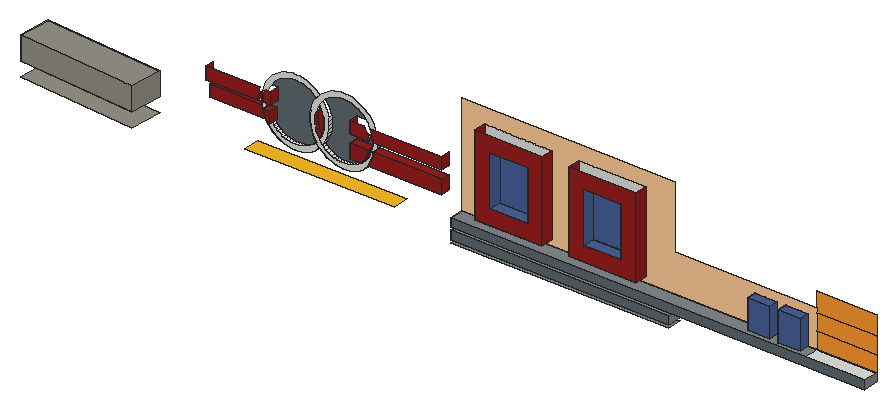
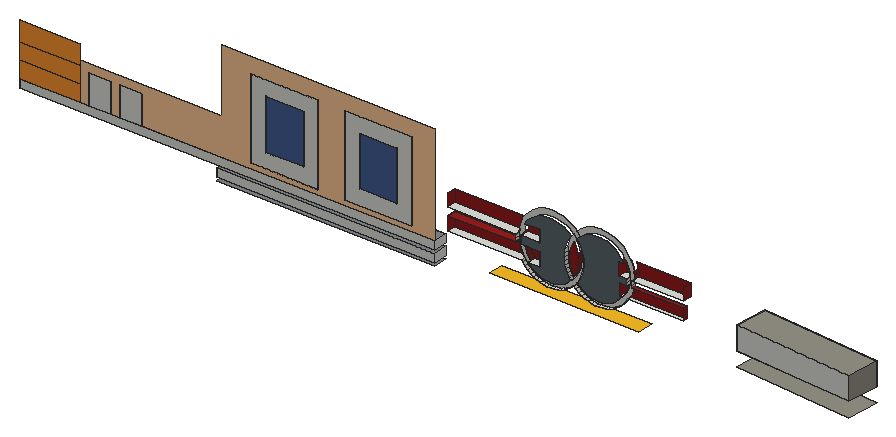
# SketchUp Ruby script. Lengths in inches.
U = 1.inch
M = Sketchup.active_model
def pt(a) = Geom::Point3d.new(a.map { |v| v * U })
def face(e, loops, mat)
  f = e.add_face(loops[0].map { |a| pt(a) })
  loops[1..].each { |l| e.add_face(l.map { |a| pt(a) }).erase! }
  f.material = f.back_material = mat if mat
  f
end
# faces: each face lists its corners as indices into pts; further lists are holes
def faces(e, pts, list, mat = nil) = list.each { |f| face(e, (f[0].is_a?(Array) ? f : [f]).map { |l| l.map { |i| pts[i] } }, mat) }
# xy, xz, yz: faces in a plane at the given z, y or x. An outline is a flat list of corners, or four numbers for a rectangle; further outlines are holes
def ring(l) = l.size == 4 ? [[l[0], l[1]], [l[2], l[1]], [l[2], l[3]], [l[0], l[3]]] : l.each_slice(2).to_a
def flat(e, list, mat, &to3) = list.each { |f| face(e, (f[0].is_a?(Array) ? f : [f]).map { |l| ring(l).map { |u, v| to3.(u, v) } }, mat) }
def xy(e, z, list, mat = nil) = flat(e, list, mat) { |x, y| [x, y, z] }
def xz(e, y, list, mat = nil) = flat(e, list, mat) { |x, z| [x, y, z] }
def yz(e, x, list, mat = nil) = flat(e, list, mat) { |y, z| [x, y, z] }
def lines(e, pts, list) = list.each { |a, b| e.add_line(pt(pts[a]), pt(pts[b])) }
# prism: a flat outline (further loops are holes) pulled along v
def prism(e, loops, v, mat = nil)
  f = face(e, loops, mat); d = Geom::Vector3d.new(v.map { |x| x * U })
  f.pushpull(f.normal.samedirection?(d) ? d.length : -d.length)
end
def box(e, o, s, mat = nil) = prism(e, [[o, [o[0] + s[0], o[1], o[2]], [o[0] + s[0], o[1] + s[1], o[2]], [o[0], o[1] + s[1], o[2]]]], [0, 0, s[2]], mat)
def at(x, y, z, deg = 0) = Geom::Transformation.translation(pt([x, y, z])) * Geom::Transformation.rotation(ORIGIN, Z_AXIS, deg.degrees)
def axes(o, x, y, z) = Geom::Transformation.new([*x, 0, *y, 0, *z, 0, *pt(o).to_a, 1])
def part(name) = M.definitions.add(name)
# library, detail: a bought-in or finely detailed component or shape, given as its bounding box
def library(name, o, s) = part(name).tap { |d| box(d.entities, o, s) }
def detail(e, o, s) = box(e.add_group.entities, o, s)
def put(e, d, t, mat = nil) = e.add_instance(d, t).tap { |i| i.material = mat if mat }
def group(e, t, mat = nil) = e.add_group.tap { |g| g.transformation = t; g.material = mat if mat }.entities
root = M.entities
M.materials.add("[0045_Goldenrod]").color = [249, 189, 36]
M.materials.add("[Blacktop Old 01]").color = [132, 136, 139]
M.materials.add("[Color A04]").color = [155, 30, 30]
M.materials.add("[Color C02]").color = [255, 204, 153]
M.materials.add("[Color C04]").color = [255, 153, 50]
M.materials.add("[Formica Blue]").color = [71, 97, 152]
M.materials.add("[Formica Graystone]").color = [149, 146, 135]
M.materials.add("[Formica Speckled Grey]").color = [94, 105, 111]
xy(root,235.375,[[253.89,85.74,386.77,94.74]],"[Blacktop Old 01]")
xy(root,237.13,[[253.89,85.74,386.77,94.74]],"[Blacktop Old 01]")
xy(root,241.27,[[72.23,70.04,73.65,89.43,1.43,94.74,0,75.36]],"[Formica Graystone]")
xy(root,242.13,[[253.89,85.74,386.77,94.74]],"[Blacktop Old 01]")
xy(root,243.23,[[129.08,85.18,220.21,94.74]],"[0045_Goldenrod]")
xy(root,243.88,[[253.89,85.74,470.23,94.74],[470.23,85.74,506.36,94.74]],"[Blacktop Old 01]")
xy(root,248.88,[[470.23,85.74,506.36,94.74],[432.49,88.8,445.99,94.74],[451.3,88.8,464.8,94.74]])
xy(root,248.88,[[253.89,85.74,470.23,85.74,470.23,94.74,464.8,94.74,464.8,88.8,451.3,88.8,451.3,94.74,445.99,94.74,445.99,88.8,432.49,88.8,432.49,94.74,253.89,94.74]],"[Blacktop Old 01]")
xy(root,250.11,[[72.23,70.04,0,75.36,1.43,94.74,73.65,89.43]])
xy(root,252.22,[[267.8,87.3,308.68,94.74],[324.8,87.3,365.68,94.74]],"[Color A04]")
xy(root,257.2,[[189.61,89.24,196.88,94.74],[200.65,89.24,245.58,94.74]])
xy(root,258.6875,[[139.59,89.24,140.74,94.74],[102.1,92.37,136.0625,94.74]])
xy(root,261.22,[[276.8,87.3,299.68,94.74],[333.8,87.3,356.68,94.74]],"[Formica Blue]")
xy(root,264.15,[[72.23,70.04,73.65,89.43,1.43,94.74,0,75.36]],"[Formica Graystone]")
xy(root,265.74,[[136.72,89.24,140.74,94.74],[189.61,89.24,200.92,94.74],[203.97,89.24,245.58,94.74],[102.1,92.37,133.7,94.74]],"[Color A04]")
xy(root,266.63,[[432.49,88.8,445.99,94.74],[451.3,88.8,464.8,94.74]],"[Formica Blue]")
xy(root,269.39,[[101.95,89.24,133.48,94.74],[136.48,89.24,141.51,94.74]])
xy(root,270.5625,[[189.67,89.24,201.09,94.74],[204.12,89.24,245.58,94.74]])
xz(root,85.74,[[253.89,237.13,386.77,242.13],[253.89,243.88,506.36,248.88]],"[Formica Speckled Grey]")
xz(root,87.3,[[[267.8,252.22,308.68,300.97],[276.8,261.22,299.68,291.97]],[[324.8,252.22,365.68,300.97],[333.8,261.22,356.68,291.97]]],"[Color A04]")
xz(root,88.8,[[432.49,248.88,445.99,266.63],[451.3,248.88,464.8,266.63]],"[Formica Blue]")
xz(root,89.24,[[189.61,257.2,196.88,257.2,197.62,258.07,198.66,259.6,199.53,261.22,200.22,262.93,200.74,264.7,200.92,265.74,189.61,265.74],[200.65,257.2,245.58,257.2,245.58,265.74,203.97,265.74,203.66,264.02,203.06,261.94,202.24,259.94,201.23,258.04],[139.59,258.6875,140.74,258.6875,140.74,265.74,136.72,265.74,136.77,265.41,137.21,263.62,137.84,261.88,138.64,260.22],[101.95,269.39,133.48,269.39,133.61,271.29,134,273.42,134.6,275.49,135.19,276.95,101.95,276.95],[136.48,269.39,141.51,269.39,141.51,276.95,138.52,276.95,138.13,276.21,137.43,274.51,136.92,272.73,136.59,270.92],
  [189.67,270.5625,201.09,270.5625,200.89,272.03,200.45,273.82,199.82,275.55,199.02,277.21,198.57,277.9375,189.67,277.9375],[204.12,270.5625,245.58,270.5625,245.58,277.9375,202,277.9375,202.59,276.72,203.32,274.6875,203.84,272.59]],"[Color A04]")
xz(root,92.37,[[153.66,248.1,155.8125,248.17,157.95,248.46,160.05,248.98,162.08,249.71,164.02,250.65,165.86,251.79,167.5625,253.11,168.84,254.33,167.97,255.23,166.89,256.625,165.6,255.38,164.14,254.25,162.58,253.28,160.92,252.47,159.18,251.85,157.39,251.41,155.5625,251.16,153.72,251.1,151.88,251.23,150.0625,251.56,148.29,252.07,146.58,252.77,144.96,253.64,143.43,254.68,142.02,255.87,140.74,257.2,139.61,258.65,139.59,258.6875,138.64,260.22,137.84,261.88,137.21,263.62,136.77,265.41,136.72,265.74,136.52,267.23,136.46,269.08,136.48,269.39,136.59,270.92,136.92,272.73,137.43,274.51,138.13,276.21,138.52,276.95,139,277.84,140.04,279.37,141.23,280.78,142.56,282.05,144.01,283.18,145.58,284.16,147.24,284.96,148.98,285.59,150.77,286.03,152.6,286.28,154.4375,286.34,156.28,286.2,158.09,285.88,159.87,285.36,161.57,284.67,163.2,283.8,164.73,282.76,166.14,281.57,166.88,280.79,167.14,281.18,168.54,282.83,168.82,283.1,168.19,283.76,166.54,285.15,164.75,286.36,162.85,287.38,160.85,288.2,158.78,288.8,156.65,289.18,154.5,289.34,152.34,289.27,150.2,288.98,148.11,288.46,146.08,287.73,144.13,286.79,142.3,285.65,140.59,284.32,139.04,282.83,137.64,281.18,136.43,279.39,135.41,277.49,135.19,276.95,134.6,275.49,134,273.42,133.61,271.29,133.48,269.39,133.46,269.14,133.53,266.98,133.7,265.74,133.82,264.84,134.34,262.75,135.07,260.72,136.01,258.77,136.0625,258.6875,137.15,256.9375,138.47,255.23,139.97,253.68,141.62,252.28,143.4,251.07,145.31,250.05,147.3,249.24,149.38,248.64,151.5,248.25],[[183.16,248.1,185.3125,248.17,187.45,248.46,189.55,248.98,191.58,249.71,193.52,250.65,195.36,251.79,197.0625,253.11,198.62,254.61,200.01,256.26,200.65,257.2,201.23,258.04,202.24,259.94,203.06,261.94,203.66,264.02,203.97,265.74,204.04,266.14,204.08,266.6,204.2,268.3,204.13,270.45,204.12,270.5625,203.84,272.59,203.32,274.6875,202.59,276.72,202,277.9375,201.65,278.66,200.51,280.5,199.19,282.2,197.69,283.76,196.04,285.15,194.25,286.36,192.35,287.38,190.35,288.2,188.28,288.8,186.15,289.18,184,289.34,181.84,289.27,179.7,288.98,177.61,288.46,175.58,287.73,173.63,286.79,171.8,285.65,170.09,284.32,168.82,283.1,168.54,282.83,167.14,281.18,166.88,280.79,165.93,279.39,164.91,277.49,164.1,275.49,163.5,273.42,163.11,271.29,162.96,269.14,163.03,266.98,163.32,264.84,163.84,262.75,164.57,260.72,165.51,258.77,166.65,256.9375,166.89,256.625,167.97,255.23,168.84,254.33,169.47,253.68,171.12,252.28,172.9,251.07,174.81,250.05,176.8,249.24,178.88,248.64,181,248.25],[183.22,251.1,181.38,251.23,179.5625,251.56,177.79,252.07,176.08,252.77,174.46,253.64,172.93,254.68,171.52,255.87,170.78,256.64,170.24,257.2,169.11,258.65,168.83,259.11,168.14,260.22,167.34,261.88,166.71,263.62,166.27,265.41,166.02,267.23,165.96,269.08,166.09,270.92,166.42,272.73,166.93,274.51,167.63,276.21,168.5,277.84,168.83,278.32,169.54,279.37,170.73,280.78,170.76,280.8125,172.06,282.05,173.51,283.18,175.08,284.16,176.74,284.96,178.48,285.59,180.27,286.03,182.1,286.28,183.9375,286.34,185.78,286.2,187.59,285.88,189.37,285.36,191.07,284.67,192.7,283.8,194.23,282.76,195.64,281.57,196.91,280.24,198.04,278.78,198.57,277.9375,199.02,277.21,199.82,275.55,200.45,273.82,200.89,272.03,201.09,270.5625,201.14,270.2,201.2,268.36,201.07,266.6,201.0625,266.52,200.92,265.74,200.74,264.7,200.22,262.93,199.53,261.22,198.66,259.6,197.62,258.07,196.88,257.2,196.43,256.66,195.1,255.38,193.64,254.25,192.08,253.28,190.42,252.47,188.68,251.85,186.89,251.41,185.0625,251.16]],[170.78,256.64,171.73,258.04,172.74,259.94,173.56,261.94,174.16,264.02,174.54,266.14,174.7,268.3,174.63,270.45,174.34,272.59,173.82,274.6875,173.09,276.72,172.15,278.66,171.01,280.5,170.76,280.8125,170.73,280.78,169.54,279.37,168.83,278.32,169.52,277.21,170.32,275.55,170.95,273.82,171.39,272.03,171.64,270.2,171.7,268.36,171.5625,266.52,171.24,264.7,170.72,262.93,170.03,261.22,169.16,259.6,168.83,259.11,169.11,258.65,170.24,257.2]])
xz(root,92.37,[[102.1,258.6875,136.0625,258.6875,136.01,258.77,135.07,260.72,134.34,262.75,133.82,264.84,133.7,265.74,102.1,265.74]],"[Color A04]")
xz(root,94.74,[[253.89,237.13,386.77,242.13],[253.89,243.88,506.36,248.88],[432.49,248.88,445.99,266.63],[451.3,248.88,464.8,266.63],[[267.8,252.22,308.68,300.97],[276.8,261.22,299.68,291.97]],
  [[324.8,252.22,365.68,300.97],[333.8,261.22,356.68,291.97]]])
xz(root,94.74,[[168.83,259.11,169.16,259.6,170.03,261.22,170.72,262.93,171.24,264.7,171.5625,266.52,171.7,268.36,171.64,270.2,171.39,272.03,170.95,273.82,170.32,275.55,169.52,277.21,168.83,278.32,168.5,277.84,167.63,276.21,166.93,274.51,166.42,272.73,166.09,270.92,165.96,269.08,166.02,267.23,166.27,265.41,166.71,263.62,167.34,261.88,168.14,260.22]],"[Color A04]")
xz(root,94.74,[[[253.89,248.88,432.49,248.88,432.49,266.63,445.99,266.63,445.99,248.88,451.3,248.88,451.3,266.63,464.8,266.63,464.8,248.88,470.23,248.88,470.23,271.875,383.64,271.875,383.64,310.29,253.89,310.29],[324.8,252.22,365.68,300.97],[267.8,252.22,308.68,300.97]]],"[Color C02]")
xz(root,94.74,[[470.23,248.88,506.36,259.02],[470.23,259.02,506.36,269.15],[470.23,269.15,506.36,280.78]],"[Color C04]")
xz(root,94.74,[[276.8,261.22,299.68,291.97],[333.8,261.22,356.68,291.97]],"[Formica Blue]")
xz(root,94.74,[[153.72,251.1,155.5625,251.16,157.39,251.41,159.18,251.85,160.92,252.47,162.58,253.28,164.14,254.25,165.6,255.38,166.89,256.625,166.65,256.9375,165.51,258.77,164.57,260.72,163.84,262.75,163.32,264.84,163.03,266.98,162.96,269.14,163.11,271.29,163.5,273.42,164.1,275.49,164.91,277.49,165.93,279.39,166.88,280.79,166.14,281.57,164.73,282.76,163.2,283.8,161.57,284.67,159.87,285.36,158.09,285.88,156.28,286.2,154.4375,286.34,152.6,286.28,150.77,286.03,148.98,285.59,147.24,284.96,145.58,284.16,144.01,283.18,142.56,282.05,141.23,280.78,140.04,279.37,139,277.84,138.52,276.95,141.51,276.95,141.51,269.39,136.48,269.39,136.46,269.08,136.52,267.23,136.72,265.74,140.74,265.74,140.74,258.6875,139.59,258.6875,139.61,258.65,140.74,257.2,142.02,255.87,143.43,254.68,144.96,253.64,146.58,252.77,148.29,252.07,150.0625,251.56,151.88,251.23],[183.22,251.1,185.0625,251.16,186.89,251.41,188.68,251.85,190.42,252.47,192.08,253.28,193.64,254.25,195.1,255.38,196.43,256.66,196.88,257.2,189.61,257.2,189.61,265.74,200.92,265.74,201.0625,266.52,201.07,266.6,201.2,268.36,201.14,270.2,201.09,270.5625,189.67,270.5625,189.67,277.9375,198.57,277.9375,198.04,278.78,196.91,280.24,195.64,281.57,194.23,282.76,192.7,283.8,191.07,284.67,189.37,285.36,187.59,285.88,185.78,286.2,183.9375,286.34,182.1,286.28,180.27,286.03,178.48,285.59,176.74,284.96,175.08,284.16,173.51,283.18,172.06,282.05,170.76,280.8125,171.01,280.5,172.15,278.66,173.09,276.72,173.82,274.6875,174.34,272.59,174.63,270.45,174.7,268.3,174.54,266.14,174.16,264.02,173.56,261.94,172.74,259.94,171.73,258.04,170.78,256.64,171.52,255.87,172.93,254.68,174.46,253.64,176.08,252.77,177.79,252.07,179.5625,251.56,181.38,251.23]],"[Formica Speckled Grey]")
yz(root,101.95,[[89.24,269.39,94.74,276.95]],"[Color A04]")
yz(root,102.1,[[92.37,258.6875,94.74,265.74]],"[Color A04]")
yz(root,140.74,[[89.24,258.6875,94.74,265.74]],"[Color A04]")
yz(root,141.51,[[89.24,269.39,94.74,276.95]],"[Color A04]")
yz(root,189.61,[[89.24,257.2,94.74,265.74]],"[Color A04]")
yz(root,189.67,[[89.24,270.5625,94.74,277.9375]],"[Color A04]")
yz(root,245.58,[[89.24,257.2,94.74,265.74],[89.24,270.5625,94.74,277.9375]],"[Color A04]")
yz(root,253.89,[[85.74,237.13,94.74,242.13],[85.74,243.88,94.74,248.88]])
yz(root,267.8,[[87.3,252.22,94.74,300.97]],"[Color A04]")
yz(root,276.8,[[87.3,261.22,94.74,291.97]],"[Formica Blue]")
yz(root,299.68,[[87.3,261.22,94.74,291.97]],"[Formica Blue]")
yz(root,308.68,[[87.3,252.22,94.74,300.97]],"[Color A04]")
yz(root,324.8,[[87.3,252.22,94.74,300.97]],"[Color A04]")
yz(root,333.8,[[87.3,261.22,94.74,291.97]],"[Formica Blue]")
yz(root,356.68,[[87.3,261.22,94.74,291.97]],"[Formica Blue]")
yz(root,365.68,[[87.3,252.22,94.74,300.97]],"[Color A04]")
yz(root,386.77,[[85.74,237.13,94.74,242.13]],"[Blacktop Old 01]")
yz(root,432.49,[[88.8,248.88,94.74,266.63]],"[Formica Blue]")
yz(root,445.99,[[88.8,248.88,94.74,266.63]],"[Formica Blue]")
yz(root,451.3,[[88.8,248.88,94.74,266.63]],"[Formica Blue]")
yz(root,464.8,[[88.8,248.88,94.74,266.63]],"[Formica Blue]")
yz(root,506.36,[[85.74,243.88,94.74,248.88]],"[Blacktop Old 01]")
p = [[151.5,94.74,248.25],[153.66,94.74,248.1],[153.66,92.37,248.1],[151.5,92.37,248.25],[155.8125,94.74,248.17],[155.8125,92.37,248.17],
  [181,94.74,248.25],[183.16,94.74,248.1],[183.16,92.37,248.1],[181,92.37,248.25],[185.3125,94.74,248.17],[185.3125,92.37,248.17],
  [157.95,94.74,248.46],[157.95,92.37,248.46],[187.45,94.74,248.46],[187.45,92.37,248.46],[149.38,94.74,248.64],[149.38,92.37,248.64],
  [178.88,94.74,248.64],[178.88,92.37,248.64],[160.05,94.74,248.98],[160.05,92.37,248.98],[189.55,94.74,248.98],[189.55,92.37,248.98],
  [147.3,94.74,249.24],[147.3,92.37,249.24],[176.8,94.74,249.24],[176.8,92.37,249.24],[162.08,94.74,249.71],[162.08,92.37,249.71],
  [191.58,94.74,249.71],[191.58,92.37,249.71],[145.31,94.74,250.05],[145.31,92.37,250.05],[174.81,94.74,250.05],[174.81,92.37,250.05],
  [164.02,94.74,250.65],[164.02,92.37,250.65],[193.52,94.74,250.65],[193.52,92.37,250.65],[72.23,70.04,264.15],[0,75.36,264.15],
  [0,75.36,250.11],[72.23,70.04,250.11],[73.65,89.43,250.11],[73.65,89.43,264.15],[1.43,94.74,264.15],[1.43,94.74,250.11],
  [143.4,94.74,251.07],[143.4,92.37,251.07],[172.9,94.74,251.07],[172.9,92.37,251.07],[165.86,94.74,251.79],[165.86,92.37,251.79],
  [195.36,94.74,251.79],[195.36,92.37,251.79],[141.62,94.74,252.28],[141.62,92.37,252.28],[153.72,94.74,251.1],[151.88,94.74,251.23],
  [151.88,92.37,251.23],[153.72,92.37,251.1],[155.5625,94.74,251.16],[155.5625,92.37,251.16],[171.12,94.74,252.28],[171.12,92.37,252.28],
  [183.22,94.74,251.1],[181.38,94.74,251.23],[181.38,92.37,251.23],[183.22,92.37,251.1],[185.0625,94.74,251.16],[185.0625,92.37,251.16],
  [150.0625,94.74,251.56],[150.0625,92.37,251.56],[157.39,94.74,251.41],[157.39,92.37,251.41],[179.5625,94.74,251.56],[179.5625,92.37,251.56],
  [186.89,94.74,251.41],[186.89,92.37,251.41],[159.18,94.74,251.85],[159.18,92.37,251.85],[188.68,94.74,251.85],[188.68,92.37,251.85],
  [148.29,94.74,252.07],[148.29,92.37,252.07],[177.79,94.74,252.07],[177.79,92.37,252.07],[160.92,94.74,252.47],[160.92,92.37,252.47],
  [167.5625,94.74,253.11],[167.5625,92.37,253.11],[190.42,94.74,252.47],[190.42,92.37,252.47],[197.0625,94.74,253.11],[197.0625,92.37,253.11],
  [146.58,94.74,252.77],[146.58,92.37,252.77],[176.08,94.74,252.77],[176.08,92.37,252.77],[139.97,94.74,253.68],[139.97,92.37,253.68],
  [169.47,94.74,253.68],[169.47,92.37,253.68],[162.58,94.74,253.28],[162.58,92.37,253.28],[192.08,94.74,253.28],[192.08,92.37,253.28],
  [144.96,94.74,253.64],[144.96,92.37,253.64],[174.46,94.74,253.64],[174.46,92.37,253.64],[168.84,94.74,254.33],[168.84,92.37,254.33],
  [198.62,94.74,254.61],[198.62,92.37,254.61],[164.14,94.74,254.25],[164.14,92.37,254.25],[193.64,94.74,254.25],[193.64,92.37,254.25],
  [143.43,94.74,254.68],[143.43,92.37,254.68],[172.93,94.74,254.68],[172.93,92.37,254.68],[138.47,94.74,255.23],[138.47,92.37,255.23],
  [165.6,94.74,255.38],[165.6,92.37,255.38],[195.1,94.74,255.38],[195.1,92.37,255.38],[200.01,94.74,256.26],[200.01,92.37,256.26],
  [142.02,94.74,255.87],[142.02,92.37,255.87],[171.52,94.74,255.87],[171.52,92.37,255.87],[137.15,94.74,256.9375],[137.15,92.37,256.9375],
  [166.89,94.74,256.625],[166.89,92.37,256.625],[196.43,94.74,256.66],[196.43,92.37,256.66],[140.74,94.74,257.2],[140.74,92.37,257.2],
  [170.78,94.74,256.64],[170.78,92.37,256.64],[200.65,94.74,257.2],[200.65,92.37,257.2],[166.65,94.74,256.9375],[166.65,92.37,256.9375],
  [171.73,94.74,258.04],[171.73,92.37,258.04],[196.88,94.74,257.2],[196.88,92.37,257.2],[136.0625,94.74,258.6875],[136.0625,92.37,258.6875],
  [165.51,94.74,258.77],[165.51,92.37,258.77],[197.62,92.37,258.07],[197.62,89.24,258.07],[196.88,89.24,257.2],[201.23,92.37,258.04],
  [200.65,89.24,257.2],[201.23,89.24,258.04],[139.61,94.74,258.65],[139.61,92.37,258.65],[202.24,92.37,259.94],[202.24,89.24,259.94],
  [172.74,94.74,259.94],[172.74,92.37,259.94],[198.66,92.37,259.6],[198.66,89.24,259.6],[138.64,92.37,260.22],[139.59,92.37,258.6875],
  [139.59,89.24,258.6875],[138.64,89.24,260.22],[139.59,94.74,258.6875],[164.57,94.74,260.72],[164.57,92.37,260.72],[168.83,94.74,259.11],
  [168.14,94.74,260.22],[168.14,92.37,260.22],[168.83,92.37,259.11],[169.16,94.74,259.6],[169.16,92.37,259.6],[199.53,92.37,261.22],
  [199.53,89.24,261.22],[170.03,94.74,261.22],[170.03,92.37,261.22],[203.06,92.37,261.94],[203.06,89.24,261.94],[173.56,94.74,261.94],
  [173.56,92.37,261.94],[137.84,92.37,261.88],[137.84,89.24,261.88],[167.34,94.74,261.88],[167.34,92.37,261.88],[163.84,94.74,262.75],
  [163.84,92.37,262.75],[200.22,92.37,262.93],[200.22,89.24,262.93],[170.72,94.74,262.93],[170.72,92.37,262.93],[137.21,92.37,263.62],
  [137.21,89.24,263.62],[203.66,92.37,264.02],[203.66,89.24,264.02],[166.71,94.74,263.62],[166.71,92.37,263.62],[174.16,94.74,264.02],
  [174.16,92.37,264.02],[163.32,94.74,264.84],[163.32,92.37,264.84],[200.74,92.37,264.7],[200.74,89.24,264.7],[171.24,94.74,264.7],
  [171.24,92.37,264.7],[136.77,92.37,265.41],[136.77,89.24,265.41],[166.27,94.74,265.41],[166.27,92.37,265.41],[203.97,92.37,265.74],
  [203.97,89.24,265.74],[174.54,94.74,266.14],[174.54,92.37,266.14],[200.92,92.37,265.74],[200.92,89.24,265.74],[171.5625,94.74,266.52],
  [171.5625,92.37,266.52],[163.03,94.74,266.98],[163.03,92.37,266.98],[136.72,92.37,265.74],[136.72,89.24,265.74],[166.02,94.74,267.23],
  [166.02,92.37,267.23],[133.53,94.74,266.98],[133.7,94.74,265.74],[133.7,92.37,265.74],[133.53,92.37,266.98],[136.72,94.74,265.74],
  [136.52,94.74,267.23],[136.52,92.37,267.23],[201.0625,94.74,266.52],[200.92,94.74,265.74],[201.0625,92.37,266.52],[203.97,94.74,265.74],
  [204.04,94.74,266.14],[204.04,92.37,266.14],[174.7,94.74,268.3],[174.7,92.37,268.3],[204.08,94.74,266.6],[204.08,92.37,266.6],
  [171.7,94.74,268.36],[171.7,92.37,268.36],[201.07,94.74,266.6],[201.07,92.37,266.6],[201.2,94.74,268.36],[201.2,92.37,268.36],
  [204.2,94.74,268.3],[204.2,92.37,268.3],[133.46,94.74,269.14],[133.46,92.37,269.14],[162.96,94.74,269.14],[162.96,92.37,269.14],
  [136.46,94.74,269.08],[136.46,92.37,269.08],[165.96,94.74,269.08],[165.96,92.37,269.08],[174.63,94.74,270.45],[174.63,92.37,270.45],
  [204.13,94.74,270.45],[204.13,92.37,270.45],[171.64,94.74,270.2],[171.64,92.37,270.2],[201.14,94.74,270.2],[201.14,92.37,270.2],
  [133.48,94.74,269.39],[133.48,92.37,269.39],[136.48,94.74,269.39],[136.48,92.37,269.39],[163.11,94.74,271.29],[163.11,92.37,271.29],
  [166.09,94.74,270.92],[166.09,92.37,270.92],[133.61,92.37,271.29],[133.61,89.24,271.29],[133.48,89.24,269.39],[136.48,89.24,269.39],
  [136.59,89.24,270.92],[136.59,92.37,270.92],[171.39,94.74,272.03],[171.39,92.37,272.03],[201.09,94.74,270.5625],[201.09,92.37,270.5625],
  [174.34,94.74,272.59],[174.34,92.37,272.59],[204.12,94.74,270.5625],[204.12,92.37,270.5625],[200.89,92.37,272.03],[200.89,89.24,272.03],
  [201.09,89.24,270.5625],[203.84,92.37,272.59],[204.12,89.24,270.5625],[203.84,89.24,272.59],[136.92,89.24,272.73],[136.92,92.37,272.73],
  [166.42,94.74,272.73],[166.42,92.37,272.73],[134,92.37,273.42],[134,89.24,273.42],[163.5,94.74,273.42],[163.5,92.37,273.42]]
faces(root,p,[[0,1,2,3],[1,4,5,2],[6,7,8,9],[7,10,11,8],[4,12,13,5],[10,14,15,11],[16,0,3,17],[18,6,9,19],
  [12,20,21,13],[14,22,23,15],[24,16,17,25],[26,18,19,27],[20,28,29,21],[22,30,31,23],[32,24,25,33],[34,26,27,35],
  [28,36,37,29],[30,38,39,31],[46,45,44,47],[48,32,33,49],[50,34,35,51],[36,52,53,37],[38,54,55,39],[56,48,49,57],
  [58,59,60,61],[62,58,61,63],[64,50,51,65],[66,67,68,69],[70,66,69,71],[59,72,73,60],[74,62,63,75],[67,76,77,68],
  [78,70,71,79],[80,74,75,81],[82,78,79,83],[72,84,85,73],[76,86,87,77],[88,80,81,89],[52,90,91,53],[92,82,83,93],
  [54,94,95,55],[84,96,97,85],[86,98,99,87],[100,56,57,101],[102,64,65,103],[104,88,89,105],[106,92,93,107],[96,108,109,97],
  [98,110,111,99],[90,112,113,91],[94,114,115,95],[116,104,105,117],[118,106,107,119],[108,120,121,109],[110,122,123,111],[124,100,101,125],
  [112,102,103,113],[126,116,117,127],[128,118,119,129],[114,130,131,115],[120,132,133,121],[122,134,135,123],[136,124,125,137],[138,126,127,139],
  [140,128,129,141],[132,142,143,133],[134,144,145,135],[130,146,147,131],[148,138,139,149],[144,150,151,145],[152,140,141,153],[154,136,137,155],
  [156,148,149,157],[142,164,165,143],[150,168,169,151],[164,176,173,165],[177,156,157,178],[168,191,192,169],[197,177,178,198],[191,209,210,192],
  [211,197,198,212],[209,223,224,210],[229,211,212,230],[235,236,237,238],[239,240,241,231],[242,243,225,244],[245,246,247,221],[223,248,249,224],
  [246,250,251,247],[254,242,244,255],[256,254,255,257],[250,258,259,251],[260,235,238,261],[262,229,230,263],[240,264,265,241],[248,268,269,249],
  [258,270,271,259],[274,256,257,275],[276,260,261,277],[264,278,279,265],[280,262,263,281],[292,274,275,293],[268,294,295,269],[270,296,297,271],
  [310,280,281,311]])
faces(root,p,[[40,41,42,43],[44,45,40,43],[46,47,42,41]],"[Formica Graystone]")
faces(root,p,[[153,158,159,160],[161,147,162,163],[166,161,163,167],[158,170,171,159],[172,173,174,175],[179,180,181,182],[183,179,182,184],[170,185,186,171],
  [187,183,184,188],[189,166,167,190],[193,172,175,194],[180,195,196,181],[185,199,200,186],[201,187,188,202],[203,193,194,204],[205,189,190,206],
  [195,207,208,196],[199,213,214,200],[215,201,202,216],[217,203,204,218],[207,219,220,208],[221,205,206,222],[213,225,226,214],[227,215,216,228],
  [231,217,218,232],[219,233,234,220],[252,227,228,253],[233,266,267,234],[272,252,253,273],[266,282,283,267],[277,284,285,286],[279,287,288,289],
  [290,272,273,291],[293,298,299,300],[301,297,302,303],[289,288,304,305],[282,306,307,283],[284,308,309,285]],"[Color A04]")
